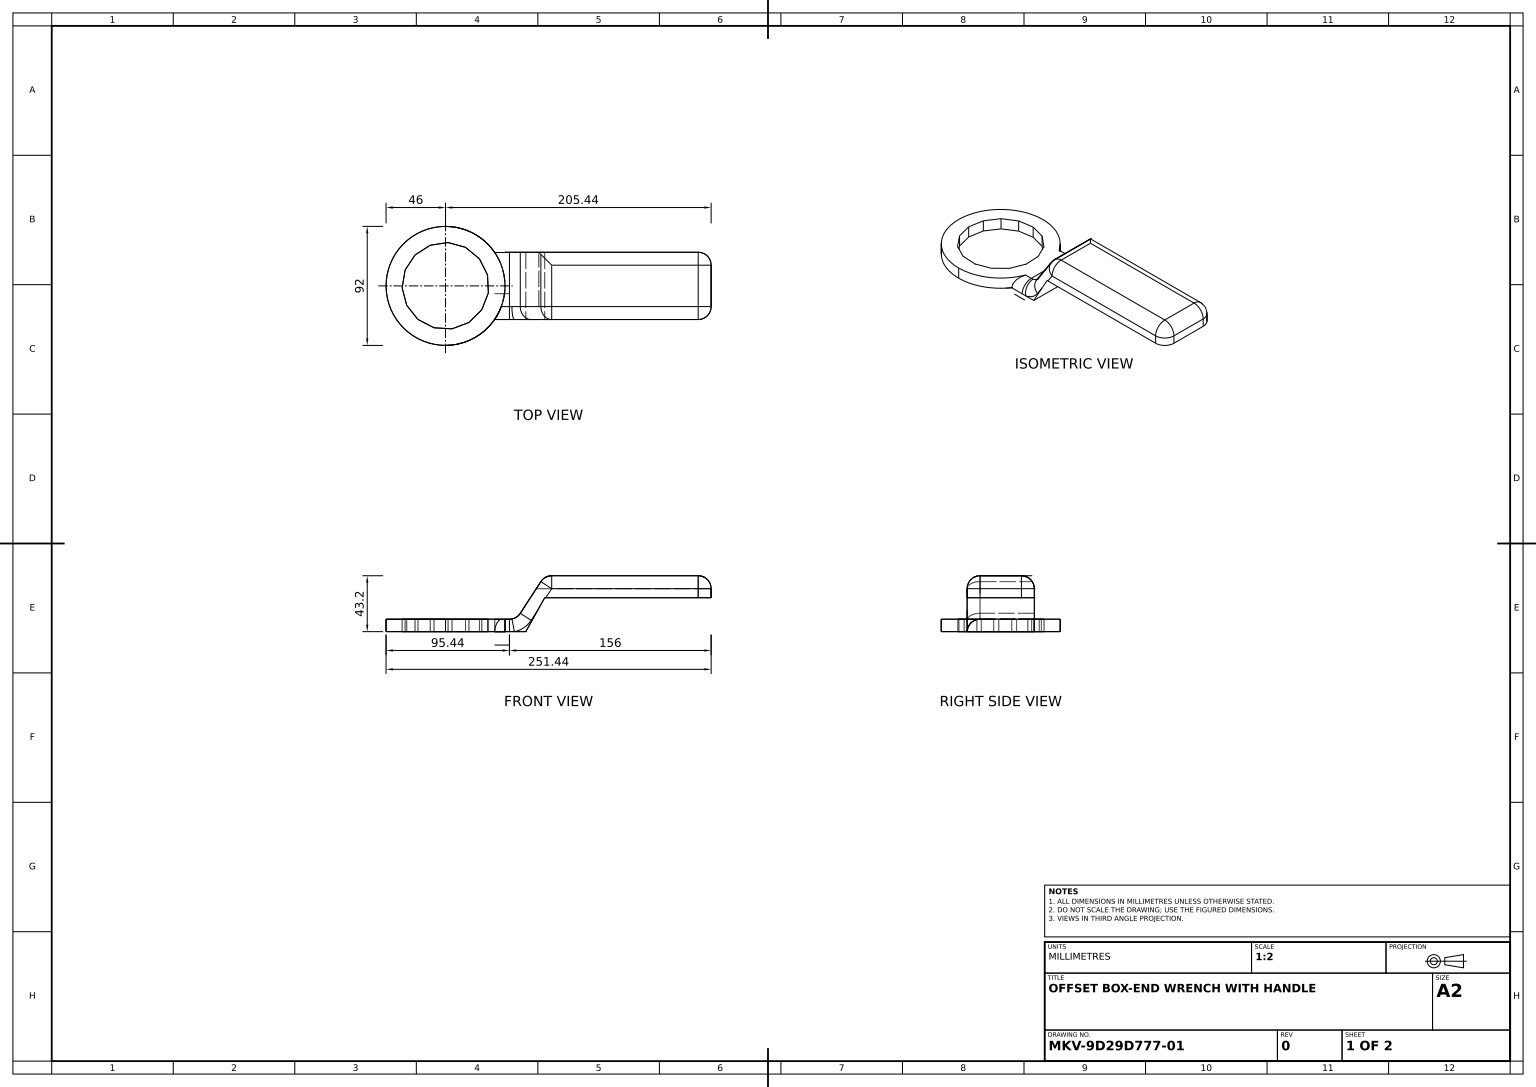
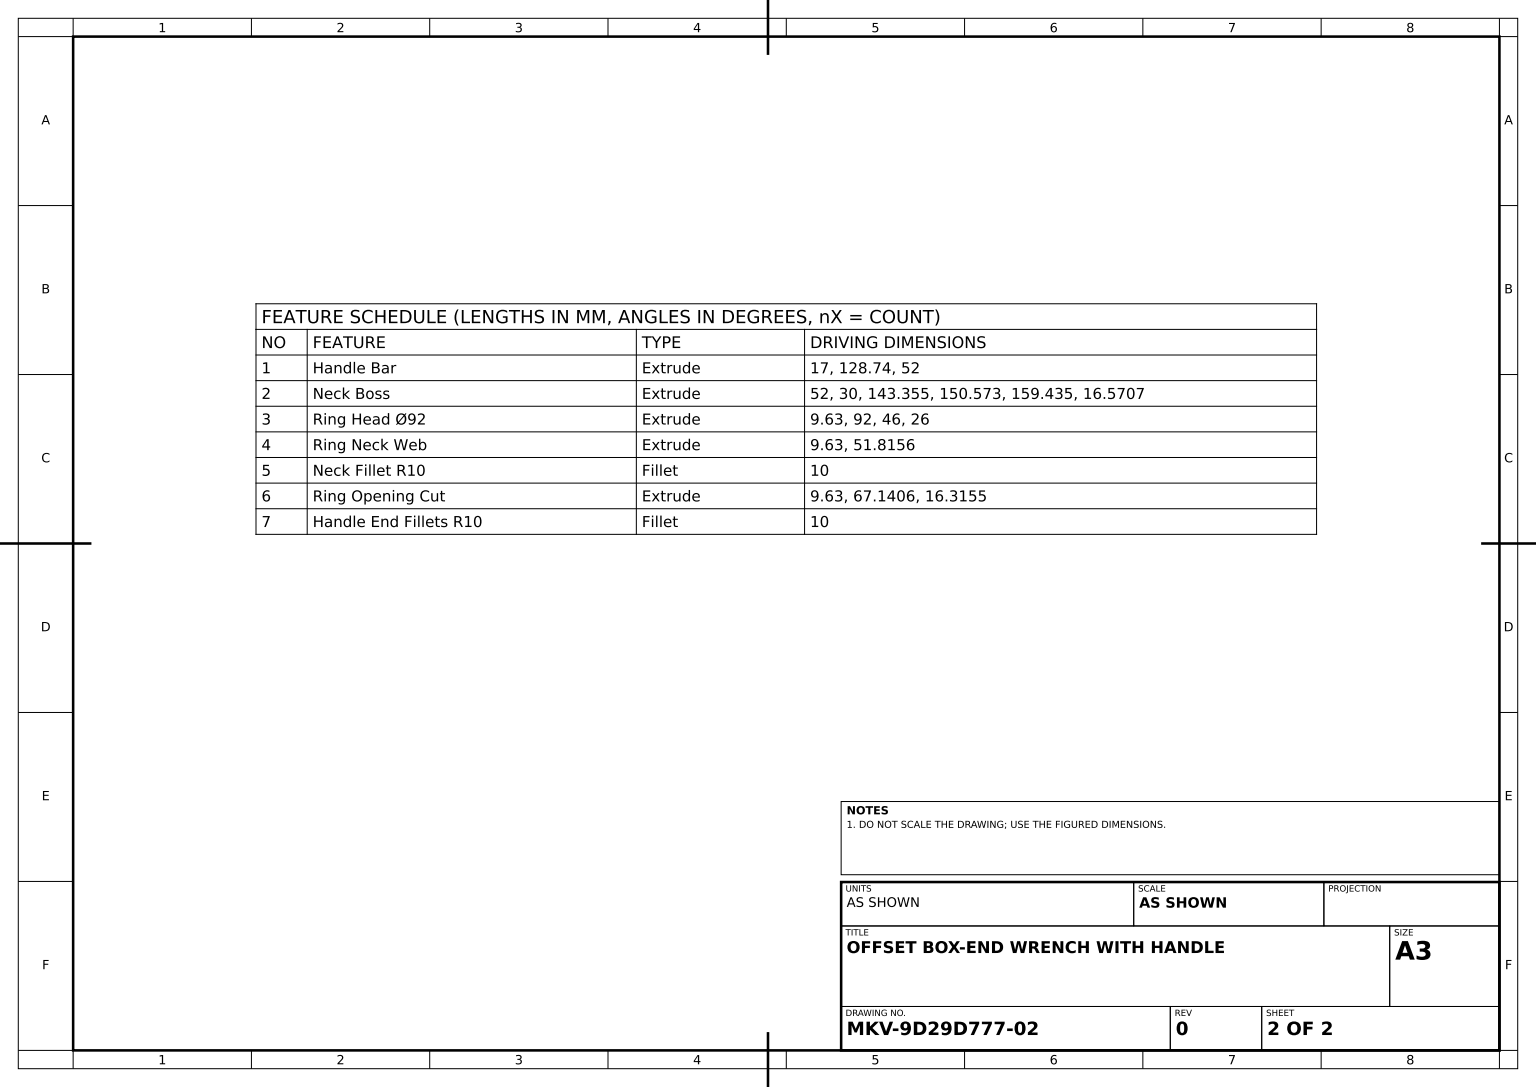
ISO-10303-21;
HEADER;
FILE_DESCRIPTION((''),'2;1');
FILE_NAME('','',(''),(''),'','','');
FILE_SCHEMA(('AUTOMOTIVE_DESIGN'));
ENDSEC;
DATA;
#1=APPLICATION_CONTEXT('');
#2=PRODUCT_CONTEXT('',#1,'mechanical');
#3=PRODUCT('','','',(#2));
#4=PRODUCT_DEFINITION_FORMATION('','',#3);
#5=PRODUCT_DEFINITION_CONTEXT('',#1,'design');
#6=PRODUCT_DEFINITION('','',#4,#5);
#7=PRODUCT_DEFINITION_SHAPE('','',#6);
#8=(LENGTH_UNIT()NAMED_UNIT(*)SI_UNIT(.MILLI.,.METRE.));
#9=(NAMED_UNIT(*)PLANE_ANGLE_UNIT()SI_UNIT($,.RADIAN.));
#10=(NAMED_UNIT(*)SI_UNIT($,.STERADIAN.)SOLID_ANGLE_UNIT());
#11=UNCERTAINTY_MEASURE_WITH_UNIT(LENGTH_MEASURE(1.E-05),#8,'distance_accuracy_value','');
#12=(GEOMETRIC_REPRESENTATION_CONTEXT(3)GLOBAL_UNCERTAINTY_ASSIGNED_CONTEXT((#11))GLOBAL_UNIT_ASSIGNED_CONTEXT((#8,#9,#10))REPRESENTATION_CONTEXT('',''));
#13=CARTESIAN_POINT('',(-87.791409,-26.199202,26.));
#14=VERTEX_POINT('',#13);
#15=CARTESIAN_POINT('',(-89.709963,-16.38497,16.));
#16=VERTEX_POINT('',#15);
#17=CARTESIAN_POINT('',(-87.791409,-26.199202,16.));
#18=DIRECTION('',(-0.981423207,-0.191855384,0.));
#19=DIRECTION('',(0.191855384,-0.981423207,0.));
#20=AXIS2_PLACEMENT_3D('',#17,#18,#19);
#21=CIRCLE('',#20,10.);
#22=EDGE_CURVE('',#14,#16,#21,.T.);
#23=ORIENTED_EDGE('',*,*,#22,.F.);
#24=CARTESIAN_POINT('',(-74.862463,-17.474841,26.));
#25=VERTEX_POINT('',#24);
#26=CARTESIAN_POINT('',(-91.628516,-6.570738,26.));
#27=DIRECTION('',(0.,0.,-1.));
#28=DIRECTION('',(-1.,0.,0.));
#29=AXIS2_PLACEMENT_3D('',#26,#27,#28);
#30=CIRCLE('',#29,20.);
#31=EDGE_CURVE('',#25,#14,#30,.T.);
#32=ORIENTED_EDGE('',*,*,#31,.F.);
#33=CARTESIAN_POINT('',(-83.24549,-12.022789,16.));
#34=VERTEX_POINT('',#33);
#35=CARTESIAN_POINT('',(-74.862463,-17.474841,16.));
#36=DIRECTION('',(-0.545205123,-0.838302674,0.));
#37=DIRECTION('',(0.838302674,-0.545205123,0.));
#38=AXIS2_PLACEMENT_3D('',#35,#36,#37);
#39=CIRCLE('',#38,10.);
#40=EDGE_CURVE('',#25,#34,#39,.T.);
#41=ORIENTED_EDGE('',*,*,#40,.T.);
#42=CARTESIAN_POINT('',(-91.628516,-6.570738,16.));
#43=DIRECTION('',(0.,0.,1.));
#44=AXIS2_PLACEMENT_3D('',#42,#43,#28);
#45=CIRCLE('',#44,10.);
#46=EDGE_CURVE('',#16,#34,#45,.T.);
#47=ORIENTED_EDGE('',*,*,#46,.F.);
#48=EDGE_LOOP('',(#23,#32,#41,#47));
#49=FACE_OUTER_BOUND('',#48,.T.);
#50=AXIS2_PLACEMENT_3D('',#42,#27,#28);
#51=TOROIDAL_SURFACE('',#50,20.,10.);
#52=ADVANCED_FACE('',(#49),#51,.T.);
#53=ORIENTED_EDGE('',*,*,#31,.T.);
#54=CARTESIAN_POINT('',(-78.985122,-26.199202,26.));
#55=VERTEX_POINT('',#54);
#56=CARTESIAN_POINT('',(0.,-26.199202,26.));
#57=DIRECTION('',(1.,0.,0.));
#58=VECTOR('',#57,1000.);
#59=LINE('',#56,#58);
#60=EDGE_CURVE('',#14,#55,#59,.T.);
#61=ORIENTED_EDGE('',*,*,#60,.T.);
#62=CARTESIAN_POINT('',(-69.631281,-9.43142,26.));
#63=VERTEX_POINT('',#62);
#64=CARTESIAN_POINT('',(-49.092725,27.386184,26.));
#65=DIRECTION('',(-0.487170738,-0.873306745,0.));
#66=VECTOR('',#65,1000.);
#67=LINE('',#64,#66);
#68=EDGE_CURVE('',#63,#55,#67,.T.);
#69=ORIENTED_EDGE('',*,*,#68,.F.);
#70=VECTOR('',#36,1000.);
#71=LINE('',#24,#70);
#72=EDGE_CURVE('',#63,#25,#71,.T.);
#73=ORIENTED_EDGE('',*,*,#72,.T.);
#74=EDGE_LOOP('',(#53,#61,#69,#73));
#75=FACE_OUTER_BOUND('',#74,.T.);
#76=CARTESIAN_POINT('',(-64.37,17.,26.));
#77=AXIS2_PLACEMENT_3D('',#76,#27,#28);
#78=PLANE('',#77);
#79=ADVANCED_FACE('',(#75),#78,.F.);
#80=CARTESIAN_POINT('',(-172.324486,-26.200738,-12.239874));
#81=VERTEX_POINT('',#80);
#82=CARTESIAN_POINT('',(-172.324486,-16.570738,-12.239874));
#83=VERTEX_POINT('',#82);
#84=DIRECTION('',(0.,1.,0.));
#85=VECTOR('',#84,1000.);
#86=LINE('',#80,#85);
#87=EDGE_CURVE('',#81,#83,#86,.T.);
#88=ORIENTED_EDGE('',*,*,#87,.T.);
#89=CARTESIAN_POINT('',(-174.600375,-16.570738,1.53266));
#90=VERTEX_POINT('',#89);
#91=DIRECTION('',(-0.163037326,0.,0.986619902));
#92=VECTOR('',#91,1000.);
#93=LINE('',#82,#92);
#94=EDGE_CURVE('',#83,#90,#93,.T.);
#95=ORIENTED_EDGE('',*,*,#94,.T.);
#96=CARTESIAN_POINT('',(-174.600375,-26.200738,1.53266));
#97=VERTEX_POINT('',#96);
#98=LINE('',#96,#85);
#99=EDGE_CURVE('',#97,#90,#98,.T.);
#100=ORIENTED_EDGE('',*,*,#99,.F.);
#101=LINE('',#80,#92);
#102=EDGE_CURVE('',#81,#97,#101,.T.);
#103=ORIENTED_EDGE('',*,*,#102,.F.);
#104=EDGE_LOOP('',(#88,#95,#100,#103));
#105=FACE_OUTER_BOUND('',#104,.T.);
#106=DIRECTION('',(-0.986619902,0.,-0.163037326));
#107=AXIS2_PLACEMENT_3D('',#80,#106,#91);
#108=PLANE('',#107);
#109=ADVANCED_FACE('',(#105),#108,.F.);
#110=CARTESIAN_POINT('',(-141.065092,-26.200738,-46.));
#111=VERTEX_POINT('',#110);
#112=CARTESIAN_POINT('',(-141.065092,-16.570738,-46.));
#113=VERTEX_POINT('',#112);
#114=LINE('',#110,#85);
#115=EDGE_CURVE('',#111,#113,#114,.T.);
#116=ORIENTED_EDGE('',*,*,#115,.F.);
#117=CARTESIAN_POINT('',(-141.065092,-26.200738,46.));
#118=VERTEX_POINT('',#117);
#119=CARTESIAN_POINT('',(-141.065092,-26.200738,0.));
#120=AXIS2_PLACEMENT_3D('',#119,#84,#43);
#121=CIRCLE('',#120,46.);
#122=EDGE_CURVE('',#111,#118,#121,.T.);
#123=ORIENTED_EDGE('',*,*,#122,.T.);
#124=CARTESIAN_POINT('',(-141.065092,-16.570738,46.));
#125=VERTEX_POINT('',#124);
#126=LINE('',#117,#85);
#127=EDGE_CURVE('',#118,#125,#126,.T.);
#128=ORIENTED_EDGE('',*,*,#127,.T.);
#129=CARTESIAN_POINT('',(-141.065092,-16.570738,0.));
#130=AXIS2_PLACEMENT_3D('',#129,#84,#43);
#131=CIRCLE('',#130,46.);
#132=EDGE_CURVE('',#113,#125,#131,.T.);
#133=ORIENTED_EDGE('',*,*,#132,.F.);
#134=EDGE_LOOP('',(#116,#123,#128,#133));
#135=FACE_OUTER_BOUND('',#134,.T.);
#136=CYLINDRICAL_SURFACE('',#120,46.);
#137=ADVANCED_FACE('',(#135),#136,.T.);
#138=CARTESIAN_POINT('',(-122.970128,-16.570738,28.276077));
#139=VERTEX_POINT('',#138);
#140=CARTESIAN_POINT('',(-113.033603,-16.570738,18.471597));
#141=VERTEX_POINT('',#140);
#142=DIRECTION('',(0.711820595,0.,-0.702361332));
#143=VECTOR('',#142,1000.);
#144=LINE('',#138,#143);
#145=EDGE_CURVE('',#139,#141,#144,.T.);
#146=ORIENTED_EDGE('',*,*,#145,.T.);
#147=CARTESIAN_POINT('',(-113.033603,-26.200738,18.471597));
#148=VERTEX_POINT('',#147);
#149=LINE('',#147,#85);
#150=EDGE_CURVE('',#148,#141,#149,.T.);
#151=ORIENTED_EDGE('',*,*,#150,.F.);
#152=CARTESIAN_POINT('',(-122.970128,-26.200738,28.276077));
#153=VERTEX_POINT('',#152);
#154=LINE('',#152,#143);
#155=EDGE_CURVE('',#153,#148,#154,.T.);
#156=ORIENTED_EDGE('',*,*,#155,.F.);
#157=LINE('',#152,#85);
#158=EDGE_CURVE('',#153,#139,#157,.T.);
#159=ORIENTED_EDGE('',*,*,#158,.T.);
#160=EDGE_LOOP('',(#146,#151,#156,#159));
#161=FACE_OUTER_BOUND('',#160,.T.);
#162=DIRECTION('',(0.702361332,0.,0.711820595));
#163=AXIS2_PLACEMENT_3D('',#152,#162,#142);
#164=PLANE('',#163);
#165=ADVANCED_FACE('',(#161),#164,.F.);
#166=CARTESIAN_POINT('',(-136.035437,-26.200738,33.191367));
#167=VERTEX_POINT('',#166);
#168=DIRECTION('',(0.935956562,0.,-0.352115485));
#169=VECTOR('',#168,1000.);
#170=LINE('',#166,#169);
#171=EDGE_CURVE('',#167,#153,#170,.T.);
#172=ORIENTED_EDGE('',*,*,#171,.F.);
#173=CARTESIAN_POINT('',(-136.035437,-16.570738,33.191367));
#174=VERTEX_POINT('',#173);
#175=LINE('',#166,#85);
#176=EDGE_CURVE('',#167,#174,#175,.T.);
#177=ORIENTED_EDGE('',*,*,#176,.T.);
#178=LINE('',#173,#169);
#179=EDGE_CURVE('',#174,#139,#178,.T.);
#180=ORIENTED_EDGE('',*,*,#179,.T.);
#181=ORIENTED_EDGE('',*,*,#158,.F.);
#182=EDGE_LOOP('',(#172,#177,#180,#181));
#183=FACE_OUTER_BOUND('',#182,.T.);
#184=DIRECTION('',(0.352115485,0.,0.935956562));
#185=AXIS2_PLACEMENT_3D('',#166,#184,#168);
#186=PLANE('',#185);
#187=ADVANCED_FACE('',(#183),#186,.F.);
#188=CARTESIAN_POINT('',(-107.943977,-16.570738,5.47321));
#189=VERTEX_POINT('',#188);
#190=CARTESIAN_POINT('',(-108.581293,-16.570738,-8.471545));
#191=VERTEX_POINT('',#190);
#192=DIRECTION('',(-0.045655243,0.,-0.998957256));
#193=VECTOR('',#192,1000.);
#194=LINE('',#188,#193);
#195=EDGE_CURVE('',#189,#191,#194,.T.);
#196=ORIENTED_EDGE('',*,*,#195,.T.);
#197=CARTESIAN_POINT('',(-108.581293,-26.200738,-8.471545));
#198=VERTEX_POINT('',#197);
#199=LINE('',#197,#85);
#200=EDGE_CURVE('',#198,#191,#199,.T.);
#201=ORIENTED_EDGE('',*,*,#200,.F.);
#202=CARTESIAN_POINT('',(-107.943977,-26.200738,5.47321));
#203=VERTEX_POINT('',#202);
#204=LINE('',#202,#193);
#205=EDGE_CURVE('',#203,#198,#204,.T.);
#206=ORIENTED_EDGE('',*,*,#205,.F.);
#207=LINE('',#202,#85);
#208=EDGE_CURVE('',#203,#189,#207,.T.);
#209=ORIENTED_EDGE('',*,*,#208,.T.);
#210=EDGE_LOOP('',(#196,#201,#206,#209));
#211=FACE_OUTER_BOUND('',#210,.T.);
#212=DIRECTION('',(0.998957256,0.,-0.045655243));
#213=AXIS2_PLACEMENT_3D('',#202,#212,#192);
#214=PLANE('',#213);
#215=ADVANCED_FACE('',(#211),#214,.F.);
#216=ORIENTED_EDGE('',*,*,#102,.T.);
#217=CARTESIAN_POINT('',(-171.077709,-26.200738,15.040183));
#218=VERTEX_POINT('',#217);
#219=DIRECTION('',(0.252352458,0.,0.967635384));
#220=VECTOR('',#219,1000.);
#221=LINE('',#96,#220);
#222=EDGE_CURVE('',#97,#218,#221,.T.);
#223=ORIENTED_EDGE('',*,*,#222,.T.);
#224=CARTESIAN_POINT('',(-162.365588,-26.200738,25.947122));
#225=VERTEX_POINT('',#224);
#226=DIRECTION('',(0.62410821,0.,0.781337918));
#227=VECTOR('',#226,1000.);
#228=LINE('',#217,#227);
#229=EDGE_CURVE('',#218,#225,#228,.T.);
#230=ORIENTED_EDGE('',*,*,#229,.T.);
#231=CARTESIAN_POINT('',(-149.970418,-26.200738,32.367567));
#232=VERTEX_POINT('',#231);
#233=DIRECTION('',(0.887949982,0.,0.459940028));
#234=VECTOR('',#233,1000.);
#235=LINE('',#224,#234);
#236=EDGE_CURVE('',#225,#232,#235,.T.);
#237=ORIENTED_EDGE('',*,*,#236,.T.);
#238=DIRECTION('',(0.998257136,0.,0.059014328));
#239=VECTOR('',#238,1000.);
#240=LINE('',#231,#239);
#241=EDGE_CURVE('',#232,#167,#240,.T.);
#242=ORIENTED_EDGE('',*,*,#241,.T.);
#243=ORIENTED_EDGE('',*,*,#171,.T.);
#244=ORIENTED_EDGE('',*,*,#155,.T.);
#245=DIRECTION('',(0.364604381,0.,-0.931162524));
#246=VECTOR('',#245,1000.);
#247=LINE('',#147,#246);
#248=EDGE_CURVE('',#148,#203,#247,.T.);
#249=ORIENTED_EDGE('',*,*,#248,.T.);
#250=ORIENTED_EDGE('',*,*,#205,.T.);
#251=CARTESIAN_POINT('',(-114.835353,-26.200738,-20.951493));
#252=VERTEX_POINT('',#251);
#253=DIRECTION('',(-0.448020661,0.,-0.894023203));
#254=VECTOR('',#253,1000.);
#255=LINE('',#197,#254);
#256=EDGE_CURVE('',#198,#252,#255,.T.);
#257=ORIENTED_EDGE('',*,*,#256,.T.);
#258=CARTESIAN_POINT('',(-125.624772,-26.200738,-29.808737));
#259=VERTEX_POINT('',#258);
#260=DIRECTION('',(-0.772919236,0.,-0.634504417));
#261=VECTOR('',#260,1000.);
#262=LINE('',#251,#261);
#263=EDGE_CURVE('',#252,#259,#262,.T.);
#264=ORIENTED_EDGE('',*,*,#263,.T.);
#265=CARTESIAN_POINT('',(-139.083964,-26.200738,-33.51178));
#266=VERTEX_POINT('',#265);
#267=DIRECTION('',(-0.964173054,0.,-0.265274052));
#268=VECTOR('',#267,1000.);
#269=LINE('',#258,#268);
#270=EDGE_CURVE('',#259,#266,#269,.T.);
#271=ORIENTED_EDGE('',*,*,#270,.T.);
#272=CARTESIAN_POINT('',(-152.88571,-26.200738,-31.420332));
#273=VERTEX_POINT('',#272);
#274=DIRECTION('',(-0.988712591,0.,0.149824606));
#275=VECTOR('',#274,1000.);
#276=LINE('',#265,#275);
#277=EDGE_CURVE('',#266,#273,#276,.T.);
#278=ORIENTED_EDGE('',*,*,#277,.T.);
#279=CARTESIAN_POINT('',(-164.643564,-26.200738,-23.896023));
#280=VERTEX_POINT('',#279);
#281=DIRECTION('',(-0.842294739,0.,0.539017228));
#282=VECTOR('',#281,1000.);
#283=LINE('',#272,#282);
#284=EDGE_CURVE('',#273,#280,#283,.T.);
#285=ORIENTED_EDGE('',*,*,#284,.T.);
#286=DIRECTION('',(-0.550236475,0.,0.835008875));
#287=VECTOR('',#286,1000.);
#288=LINE('',#279,#287);
#289=EDGE_CURVE('',#280,#81,#288,.T.);
#290=ORIENTED_EDGE('',*,*,#289,.T.);
#291=EDGE_LOOP('',(#216,#223,#230,#237,#242,#243,#244,#249,#250,#257,#264,#271,#278,#285,#290));
#292=FACE_BOUND('',#291,.T.);
#293=EDGE_CURVE('',#118,#111,#121,.T.);
#294=ORIENTED_EDGE('',*,*,#293,.F.);
#295=ORIENTED_EDGE('',*,*,#122,.F.);
#296=EDGE_LOOP('',(#294,#295));
#297=FACE_OUTER_BOUND('',#296,.T.);
#298=PLANE('',#120);
#299=ADVANCED_FACE('',(#292,#297),#298,.F.);
#300=CARTESIAN_POINT('',(-152.88571,-16.570738,-31.420332));
#301=VERTEX_POINT('',#300);
#302=LINE('',#272,#85);
#303=EDGE_CURVE('',#273,#301,#302,.T.);
#304=ORIENTED_EDGE('',*,*,#303,.F.);
#305=ORIENTED_EDGE('',*,*,#277,.F.);
#306=CARTESIAN_POINT('',(-139.083964,-16.570738,-33.51178));
#307=VERTEX_POINT('',#306);
#308=LINE('',#265,#85);
#309=EDGE_CURVE('',#266,#307,#308,.T.);
#310=ORIENTED_EDGE('',*,*,#309,.T.);
#311=LINE('',#306,#275);
#312=EDGE_CURVE('',#307,#301,#311,.T.);
#313=ORIENTED_EDGE('',*,*,#312,.T.);
#314=EDGE_LOOP('',(#304,#305,#310,#313));
#315=FACE_OUTER_BOUND('',#314,.T.);
#316=DIRECTION('',(-0.149824606,0.,-0.988712591));
#317=AXIS2_PLACEMENT_3D('',#265,#316,#274);
#318=PLANE('',#317);
#319=ADVANCED_FACE('',(#315),#318,.F.);
#320=CARTESIAN_POINT('',(64.37,7.,16.));
#321=VERTEX_POINT('',#320);
#322=CARTESIAN_POINT('',(54.37,17.,16.));
#323=VERTEX_POINT('',#322);
#324=CARTESIAN_POINT('',(54.37,7.,16.));
#325=AXIS2_PLACEMENT_3D('',#324,#43,#57);
#326=CIRCLE('',#325,10.);
#327=EDGE_CURVE('',#321,#323,#326,.T.);
#328=ORIENTED_EDGE('',*,*,#327,.T.);
#329=CARTESIAN_POINT('',(54.37,7.,26.));
#330=VERTEX_POINT('',#329);
#331=AXIS2_PLACEMENT_3D('',#324,#28,#27);
#332=CIRCLE('',#331,10.);
#333=EDGE_CURVE('',#330,#323,#332,.T.);
#334=ORIENTED_EDGE('',*,*,#333,.F.);
#335=AXIS2_PLACEMENT_3D('',#324,#84,#43);
#336=CIRCLE('',#335,10.);
#337=EDGE_CURVE('',#330,#321,#336,.T.);
#338=ORIENTED_EDGE('',*,*,#337,.T.);
#339=EDGE_LOOP('',(#328,#334,#338));
#340=FACE_OUTER_BOUND('',#339,.T.);
#341=AXIS2_PLACEMENT_3D('',#324,#84,#57);
#342=SPHERICAL_SURFACE('',#341,10.);
#343=ADVANCED_FACE('',(#340),#342,.T.);
#344=ORIENTED_EDGE('',*,*,#208,.F.);
#345=ORIENTED_EDGE('',*,*,#248,.F.);
#346=ORIENTED_EDGE('',*,*,#150,.T.);
#347=LINE('',#140,#246);
#348=EDGE_CURVE('',#141,#189,#347,.T.);
#349=ORIENTED_EDGE('',*,*,#348,.T.);
#350=EDGE_LOOP('',(#344,#345,#346,#349));
#351=FACE_OUTER_BOUND('',#350,.T.);
#352=DIRECTION('',(0.931162524,0.,0.364604381));
#353=AXIS2_PLACEMENT_3D('',#147,#352,#245);
#354=PLANE('',#353);
#355=ADVANCED_FACE('',(#351),#354,.F.);
#356=CARTESIAN_POINT('',(-114.835353,-16.570738,-20.951493));
#357=VERTEX_POINT('',#356);
#358=LINE('',#251,#85);
#359=EDGE_CURVE('',#252,#357,#358,.T.);
#360=ORIENTED_EDGE('',*,*,#359,.F.);
#361=ORIENTED_EDGE('',*,*,#256,.F.);
#362=ORIENTED_EDGE('',*,*,#200,.T.);
#363=LINE('',#190,#254);
#364=EDGE_CURVE('',#191,#357,#363,.T.);
#365=ORIENTED_EDGE('',*,*,#364,.T.);
#366=EDGE_LOOP('',(#360,#361,#362,#365));
#367=FACE_OUTER_BOUND('',#366,.T.);
#368=DIRECTION('',(0.894023203,0.,-0.448020661));
#369=AXIS2_PLACEMENT_3D('',#197,#368,#253);
#370=PLANE('',#369);
#371=ADVANCED_FACE('',(#367),#370,.F.);
#372=CARTESIAN_POINT('',(64.37,0.,16.));
#373=VERTEX_POINT('',#372);
#374=CARTESIAN_POINT('',(54.37,0.,26.));
#375=VERTEX_POINT('',#374);
#376=CARTESIAN_POINT('',(54.37,0.,16.));
#377=DIRECTION('',(0.,-1.,0.));
#378=AXIS2_PLACEMENT_3D('',#376,#377,#27);
#379=CIRCLE('',#378,10.);
#380=EDGE_CURVE('',#373,#375,#379,.T.);
#381=ORIENTED_EDGE('',*,*,#380,.F.);
#382=CARTESIAN_POINT('',(64.37,17.,16.));
#383=VECTOR('',#377,1000.);
#384=LINE('',#382,#383);
#385=EDGE_CURVE('',#321,#373,#384,.T.);
#386=ORIENTED_EDGE('',*,*,#385,.F.);
#387=ORIENTED_EDGE('',*,*,#337,.F.);
#388=CARTESIAN_POINT('',(54.37,17.,26.));
#389=LINE('',#388,#85);
#390=EDGE_CURVE('',#375,#330,#389,.T.);
#391=ORIENTED_EDGE('',*,*,#390,.F.);
#392=EDGE_LOOP('',(#381,#386,#387,#391));
#393=FACE_OUTER_BOUND('',#392,.T.);
#394=AXIS2_PLACEMENT_3D('',#322,#377,#27);
#395=CYLINDRICAL_SURFACE('',#394,10.);
#396=ADVANCED_FACE('',(#393),#395,.T.);
#397=CARTESIAN_POINT('',(-91.628516,-16.570738,-26.));
#398=VERTEX_POINT('',#397);
#399=CARTESIAN_POINT('',(-95.065092,-16.570738,-26.));
#400=VERTEX_POINT('',#399);
#401=CARTESIAN_POINT('',(0.,-16.570738,-26.));
#402=VECTOR('',#28,1000.);
#403=LINE('',#401,#402);
#404=EDGE_CURVE('',#398,#400,#403,.T.);
#405=ORIENTED_EDGE('',*,*,#404,.T.);
#406=CARTESIAN_POINT('',(-95.065092,-16.570738,-25.815581));
#407=VERTEX_POINT('',#406);
#408=VECTOR('',#43,1000.);
#409=LINE('',#399,#408);
#410=EDGE_CURVE('',#400,#407,#409,.T.);
#411=ORIENTED_EDGE('',*,*,#410,.T.);
#412=CARTESIAN_POINT('',(-102.99206,-16.570738,-25.815581));
#413=VERTEX_POINT('',#412);
#414=CARTESIAN_POINT('',(-104.695092,-16.570738,-25.815581));
#415=LINE('',#414,#58);
#416=EDGE_CURVE('',#413,#407,#415,.T.);
#417=ORIENTED_EDGE('',*,*,#416,.F.);
#418=EDGE_CURVE('',#413,#113,#131,.T.);
#419=ORIENTED_EDGE('',*,*,#418,.T.);
#420=ORIENTED_EDGE('',*,*,#132,.T.);
#421=CARTESIAN_POINT('',(-97.939937,-16.570738,16.006904));
#422=VERTEX_POINT('',#421);
#423=EDGE_CURVE('',#125,#422,#131,.T.);
#424=ORIENTED_EDGE('',*,*,#423,.T.);
#425=CARTESIAN_POINT('',(-91.628516,-16.570738,16.006904));
#426=VERTEX_POINT('',#425);
#427=LINE('',#425,#58);
#428=EDGE_CURVE('',#422,#426,#427,.T.);
#429=ORIENTED_EDGE('',*,*,#428,.T.);
#430=VECTOR('',#27,1000.);
#431=LINE('',#397,#430);
#432=EDGE_CURVE('',#426,#398,#431,.T.);
#433=ORIENTED_EDGE('',*,*,#432,.T.);
#434=EDGE_LOOP('',(#405,#411,#417,#419,#420,#424,#429,#433));
#435=FACE_OUTER_BOUND('',#434,.T.);
#436=ORIENTED_EDGE('',*,*,#145,.F.);
#437=ORIENTED_EDGE('',*,*,#179,.F.);
#438=CARTESIAN_POINT('',(-149.970418,-16.570738,32.367567));
#439=VERTEX_POINT('',#438);
#440=LINE('',#438,#239);
#441=EDGE_CURVE('',#439,#174,#440,.T.);
#442=ORIENTED_EDGE('',*,*,#441,.F.);
#443=CARTESIAN_POINT('',(-162.365588,-16.570738,25.947122));
#444=VERTEX_POINT('',#443);
#445=LINE('',#443,#234);
#446=EDGE_CURVE('',#444,#439,#445,.T.);
#447=ORIENTED_EDGE('',*,*,#446,.F.);
#448=CARTESIAN_POINT('',(-171.077709,-16.570738,15.040183));
#449=VERTEX_POINT('',#448);
#450=LINE('',#448,#227);
#451=EDGE_CURVE('',#449,#444,#450,.T.);
#452=ORIENTED_EDGE('',*,*,#451,.F.);
#453=LINE('',#89,#220);
#454=EDGE_CURVE('',#90,#449,#453,.T.);
#455=ORIENTED_EDGE('',*,*,#454,.F.);
#456=ORIENTED_EDGE('',*,*,#94,.F.);
#457=CARTESIAN_POINT('',(-164.643564,-16.570738,-23.896023));
#458=VERTEX_POINT('',#457);
#459=LINE('',#457,#287);
#460=EDGE_CURVE('',#458,#83,#459,.T.);
#461=ORIENTED_EDGE('',*,*,#460,.F.);
#462=LINE('',#300,#282);
#463=EDGE_CURVE('',#301,#458,#462,.T.);
#464=ORIENTED_EDGE('',*,*,#463,.F.);
#465=ORIENTED_EDGE('',*,*,#312,.F.);
#466=CARTESIAN_POINT('',(-125.624772,-16.570738,-29.808737));
#467=VERTEX_POINT('',#466);
#468=LINE('',#466,#268);
#469=EDGE_CURVE('',#467,#307,#468,.T.);
#470=ORIENTED_EDGE('',*,*,#469,.F.);
#471=LINE('',#356,#261);
#472=EDGE_CURVE('',#357,#467,#471,.T.);
#473=ORIENTED_EDGE('',*,*,#472,.F.);
#474=ORIENTED_EDGE('',*,*,#364,.F.);
#475=ORIENTED_EDGE('',*,*,#195,.F.);
#476=ORIENTED_EDGE('',*,*,#348,.F.);
#477=EDGE_LOOP('',(#436,#437,#442,#447,#452,#455,#456,#461,#464,#465,#470,#473,#474,#475,#476));
#478=FACE_BOUND('',#477,.T.);
#479=AXIS2_PLACEMENT_3D('',#401,#84,#43);
#480=PLANE('',#479);
#481=ADVANCED_FACE('',(#435,#478),#480,.T.);
#482=CARTESIAN_POINT('',(-95.065092,-26.199202,-26.));
#483=VERTEX_POINT('',#482);
#484=CARTESIAN_POINT('',(-95.065092,-26.199202,-25.815581));
#485=VERTEX_POINT('',#484);
#486=LINE('',#482,#408);
#487=EDGE_CURVE('',#483,#485,#486,.T.);
#488=ORIENTED_EDGE('',*,*,#487,.T.);
#489=LINE('',#406,#383);
#490=EDGE_CURVE('',#407,#485,#489,.T.);
#491=ORIENTED_EDGE('',*,*,#490,.F.);
#492=ORIENTED_EDGE('',*,*,#410,.F.);
#493=CARTESIAN_POINT('',(-95.065092,0.,-26.));
#494=LINE('',#493,#383);
#495=EDGE_CURVE('',#400,#483,#494,.T.);
#496=ORIENTED_EDGE('',*,*,#495,.T.);
#497=EDGE_LOOP('',(#488,#491,#492,#496));
#498=FACE_OUTER_BOUND('',#497,.T.);
#499=AXIS2_PLACEMENT_3D('',#493,#28,#43);
#500=PLANE('',#499);
#501=ADVANCED_FACE('',(#498),#500,.T.);
#502=ORIENTED_EDGE('',*,*,#68,.T.);
#503=CARTESIAN_POINT('',(-78.985122,-26.199202,-26.));
#504=VERTEX_POINT('',#503);
#505=LINE('',#503,#408);
#506=EDGE_CURVE('',#504,#55,#505,.T.);
#507=ORIENTED_EDGE('',*,*,#506,.F.);
#508=CARTESIAN_POINT('',(-64.37,0.,-26.));
#509=VERTEX_POINT('',#508);
#510=CARTESIAN_POINT('',(-49.092725,27.386184,-26.));
#511=LINE('',#510,#66);
#512=EDGE_CURVE('',#509,#504,#511,.T.);
#513=ORIENTED_EDGE('',*,*,#512,.F.);
#514=CARTESIAN_POINT('',(-64.37,0.,25.973209));
#515=VERTEX_POINT('',#514);
#516=CARTESIAN_POINT('',(-64.37,0.,26.));
#517=LINE('',#516,#408);
#518=EDGE_CURVE('',#509,#515,#517,.T.);
#519=ORIENTED_EDGE('',*,*,#518,.T.);
#520=CARTESIAN_POINT('',(-66.121016,-3.138888,25.991066));
#521=CARTESIAN_POINT('',(-67.87556,-6.2841,26.));
#522=(BOUNDED_CURVE()B_SPLINE_CURVE(3,(#514,#520,#521,#62),.UNSPECIFIED.,.F.,.T.)B_SPLINE_CURVE_WITH_KNOTS((4,4),(1.497579638,1.570796327),.UNSPECIFIED.)CURVE()GEOMETRIC_REPRESENTATION_ITEM()RATIONAL_B_SPLINE_CURVE((1.,0.999553326,0.999553326,1.))REPRESENTATION_ITEM(''));
#523=EDGE_CURVE('',#515,#63,#522,.T.);
#524=ORIENTED_EDGE('',*,*,#523,.T.);
#525=EDGE_LOOP('',(#502,#507,#513,#519,#524));
#526=FACE_OUTER_BOUND('',#525,.T.);
#527=DIRECTION('',(-0.873306745,0.487170738,0.));
#528=AXIS2_PLACEMENT_3D('',#510,#527,#65);
#529=PLANE('',#528);
#530=ADVANCED_FACE('',(#526),#529,.F.);
#531=CARTESIAN_POINT('',(64.37,7.,-16.));
#532=VERTEX_POINT('',#531);
#533=CARTESIAN_POINT('',(54.37,17.,-16.));
#534=VERTEX_POINT('',#533);
#535=CARTESIAN_POINT('',(54.37,7.,-16.));
#536=AXIS2_PLACEMENT_3D('',#535,#43,#28);
#537=CIRCLE('',#536,10.);
#538=EDGE_CURVE('',#532,#534,#537,.T.);
#539=ORIENTED_EDGE('',*,*,#538,.F.);
#540=CARTESIAN_POINT('',(54.37,7.,-26.));
#541=VERTEX_POINT('',#540);
#542=AXIS2_PLACEMENT_3D('',#535,#84,#43);
#543=CIRCLE('',#542,10.);
#544=EDGE_CURVE('',#532,#541,#543,.T.);
#545=ORIENTED_EDGE('',*,*,#544,.T.);
#546=AXIS2_PLACEMENT_3D('',#535,#28,#84);
#547=CIRCLE('',#546,10.);
#548=EDGE_CURVE('',#534,#541,#547,.T.);
#549=ORIENTED_EDGE('',*,*,#548,.F.);
#550=EDGE_LOOP('',(#539,#545,#549));
#551=FACE_OUTER_BOUND('',#550,.T.);
#552=AXIS2_PLACEMENT_3D('',#535,#84,#57);
#553=SPHERICAL_SURFACE('',#552,10.);
#554=ADVANCED_FACE('',(#551),#553,.T.);
#555=ORIENTED_EDGE('',*,*,#446,.T.);
#556=LINE('',#231,#85);
#557=EDGE_CURVE('',#232,#439,#556,.T.);
#558=ORIENTED_EDGE('',*,*,#557,.F.);
#559=ORIENTED_EDGE('',*,*,#236,.F.);
#560=LINE('',#224,#85);
#561=EDGE_CURVE('',#225,#444,#560,.T.);
#562=ORIENTED_EDGE('',*,*,#561,.T.);
#563=EDGE_LOOP('',(#555,#558,#559,#562));
#564=FACE_OUTER_BOUND('',#563,.T.);
#565=DIRECTION('',(-0.459940028,0.,0.887949982));
#566=AXIS2_PLACEMENT_3D('',#224,#565,#233);
#567=PLANE('',#566);
#568=ADVANCED_FACE('',(#564),#567,.F.);
#569=CARTESIAN_POINT('',(-83.24549,-12.022789,-26.));
#570=VERTEX_POINT('',#569);
#571=CARTESIAN_POINT('',(-83.24549,-12.022789,26.));
#572=LINE('',#571,#408);
#573=EDGE_CURVE('',#570,#34,#572,.T.);
#574=ORIENTED_EDGE('',*,*,#573,.F.);
#575=CARTESIAN_POINT('',(-91.628516,-6.570738,-26.));
#576=AXIS2_PLACEMENT_3D('',#575,#43,#57);
#577=CIRCLE('',#576,10.);
#578=EDGE_CURVE('',#398,#570,#577,.T.);
#579=ORIENTED_EDGE('',*,*,#578,.F.);
#580=ORIENTED_EDGE('',*,*,#432,.F.);
#581=CARTESIAN_POINT('',(-90.982994,-16.570738,16.006904));
#582=CARTESIAN_POINT('',(-90.343493,-16.508817,16.));
#583=B_SPLINE_CURVE_WITH_KNOTS('',3,(#425,#581,#582,#15),.UNSPECIFIED.,.F.,.F.,(4,4),(0.,0.001927539),.UNSPECIFIED.);
#584=EDGE_CURVE('',#426,#16,#583,.T.);
#585=ORIENTED_EDGE('',*,*,#584,.T.);
#586=ORIENTED_EDGE('',*,*,#46,.T.);
#587=EDGE_LOOP('',(#574,#579,#580,#585,#586));
#588=FACE_OUTER_BOUND('',#587,.T.);
#589=AXIS2_PLACEMENT_3D('',#575,#27,#28);
#590=CYLINDRICAL_SURFACE('',#589,10.);
#591=ADVANCED_FACE('',(#588),#590,.F.);
#592=CARTESIAN_POINT('',(-102.99206,-26.199202,-25.815581));
#593=VERTEX_POINT('',#592);
#594=CARTESIAN_POINT('',(-103.11776,-26.199202,26.));
#595=VERTEX_POINT('',#594);
#596=CARTESIAN_POINT('',(-141.065092,-26.199202,0.));
#597=AXIS2_PLACEMENT_3D('',#596,#377,#27);
#598=CIRCLE('',#597,46.);
#599=EDGE_CURVE('',#593,#595,#598,.T.);
#600=ORIENTED_EDGE('',*,*,#599,.F.);
#601=CARTESIAN_POINT('',(-104.695092,-26.199202,-25.815581));
#602=LINE('',#601,#58);
#603=EDGE_CURVE('',#593,#485,#602,.T.);
#604=ORIENTED_EDGE('',*,*,#603,.T.);
#605=ORIENTED_EDGE('',*,*,#487,.F.);
#606=CARTESIAN_POINT('',(0.,-26.199202,-26.));
#607=LINE('',#606,#58);
#608=EDGE_CURVE('',#483,#504,#607,.T.);
#609=ORIENTED_EDGE('',*,*,#608,.T.);
#610=ORIENTED_EDGE('',*,*,#506,.T.);
#611=ORIENTED_EDGE('',*,*,#60,.F.);
#612=CARTESIAN_POINT('',(-91.628516,-26.199202,26.));
#613=VERTEX_POINT('',#612);
#614=EDGE_CURVE('',#613,#14,#59,.T.);
#615=ORIENTED_EDGE('',*,*,#614,.F.);
#616=EDGE_CURVE('',#595,#613,#59,.T.);
#617=ORIENTED_EDGE('',*,*,#616,.F.);
#618=EDGE_LOOP('',(#600,#604,#605,#609,#610,#611,#615,#617));
#619=FACE_OUTER_BOUND('',#618,.T.);
#620=AXIS2_PLACEMENT_3D('',#606,#377,#27);
#621=PLANE('',#620);
#622=ADVANCED_FACE('',(#619),#621,.T.);
#623=ORIENTED_EDGE('',*,*,#99,.T.);
#624=ORIENTED_EDGE('',*,*,#454,.T.);
#625=LINE('',#217,#85);
#626=EDGE_CURVE('',#218,#449,#625,.T.);
#627=ORIENTED_EDGE('',*,*,#626,.F.);
#628=ORIENTED_EDGE('',*,*,#222,.F.);
#629=EDGE_LOOP('',(#623,#624,#627,#628));
#630=FACE_OUTER_BOUND('',#629,.T.);
#631=DIRECTION('',(-0.967635384,0.,0.252352458));
#632=AXIS2_PLACEMENT_3D('',#96,#631,#219);
#633=PLANE('',#632);
#634=ADVANCED_FACE('',(#630),#633,.F.);
#635=ORIENTED_EDGE('',*,*,#469,.T.);
#636=ORIENTED_EDGE('',*,*,#309,.F.);
#637=ORIENTED_EDGE('',*,*,#270,.F.);
#638=LINE('',#258,#85);
#639=EDGE_CURVE('',#259,#467,#638,.T.);
#640=ORIENTED_EDGE('',*,*,#639,.T.);
#641=EDGE_LOOP('',(#635,#636,#637,#640));
#642=FACE_OUTER_BOUND('',#641,.T.);
#643=DIRECTION('',(0.265274052,0.,-0.964173054));
#644=AXIS2_PLACEMENT_3D('',#258,#643,#267);
#645=PLANE('',#644);
#646=ADVANCED_FACE('',(#642),#645,.F.);
#647=CARTESIAN_POINT('',(-58.944813,7.,26.));
#648=VERTEX_POINT('',#647);
#649=CARTESIAN_POINT('',(-58.944813,17.,16.));
#650=VERTEX_POINT('',#649);
#651=CARTESIAN_POINT('',(-58.944813,7.,16.));
#652=AXIS2_PLACEMENT_3D('',#651,#28,#377);
#653=CIRCLE('',#652,10.);
#654=EDGE_CURVE('',#648,#650,#653,.T.);
#655=ORIENTED_EDGE('',*,*,#654,.T.);
#656=CARTESIAN_POINT('',(-67.32784,12.452051,16.));
#657=VERTEX_POINT('',#656);
#658=AXIS2_PLACEMENT_3D('',#651,#43,#57);
#659=CIRCLE('',#658,10.);
#660=EDGE_CURVE('',#650,#657,#659,.T.);
#661=ORIENTED_EDGE('',*,*,#660,.T.);
#662=DIRECTION('',(-0.838302674,0.545205123,0.));
#663=AXIS2_PLACEMENT_3D('',#651,#36,#662);
#664=CIRCLE('',#663,10.);
#665=EDGE_CURVE('',#648,#657,#664,.T.);
#666=ORIENTED_EDGE('',*,*,#665,.F.);
#667=EDGE_LOOP('',(#655,#661,#666));
#668=FACE_OUTER_BOUND('',#667,.T.);
#669=AXIS2_PLACEMENT_3D('',#651,#84,#57);
#670=SPHERICAL_SURFACE('',#669,10.);
#671=ADVANCED_FACE('',(#668),#670,.T.);
#672=ORIENTED_EDGE('',*,*,#573,.T.);
#673=CARTESIAN_POINT('',(-64.37,17.,16.));
#674=DIRECTION('',(0.545205123,0.838302674,0.));
#675=VECTOR('',#674,1000.);
#676=LINE('',#673,#675);
#677=EDGE_CURVE('',#34,#657,#676,.T.);
#678=ORIENTED_EDGE('',*,*,#677,.T.);
#679=CARTESIAN_POINT('',(-67.32784,12.452051,-24.383027));
#680=VERTEX_POINT('',#679);
#681=CARTESIAN_POINT('',(-67.32784,12.452051,-26.));
#682=LINE('',#681,#430);
#683=EDGE_CURVE('',#657,#680,#682,.T.);
#684=ORIENTED_EDGE('',*,*,#683,.T.);
#685=CARTESIAN_POINT('',(-70.873679,7.,-26.));
#686=VERTEX_POINT('',#685);
#687=CARTESIAN_POINT('',(-68.390571,10.818006,-25.445758));
#688=CARTESIAN_POINT('',(-69.605961,8.949231,-26.));
#689=(BOUNDED_CURVE()B_SPLINE_CURVE(3,(#679,#687,#688,#685),.UNSPECIFIED.,.F.,.F.)B_SPLINE_CURVE_WITH_KNOTS((4,4),(4.135755197,4.71238898),.UNSPECIFIED.)CURVE()GEOMETRIC_REPRESENTATION_ITEM()RATIONAL_B_SPLINE_CURVE((1.,0.972482538,0.972482538,1.))REPRESENTATION_ITEM(''));
#690=EDGE_CURVE('',#680,#686,#689,.T.);
#691=ORIENTED_EDGE('',*,*,#690,.T.);
#692=CARTESIAN_POINT('',(-53.005903,34.473336,-26.));
#693=LINE('',#692,#70);
#694=EDGE_CURVE('',#686,#570,#693,.T.);
#695=ORIENTED_EDGE('',*,*,#694,.T.);
#696=EDGE_LOOP('',(#672,#678,#684,#691,#695));
#697=FACE_OUTER_BOUND('',#696,.T.);
#698=AXIS2_PLACEMENT_3D('',#692,#662,#36);
#699=PLANE('',#698);
#700=ADVANCED_FACE('',(#697),#699,.T.);
#701=ORIENTED_EDGE('',*,*,#229,.F.);
#702=ORIENTED_EDGE('',*,*,#626,.T.);
#703=ORIENTED_EDGE('',*,*,#451,.T.);
#704=ORIENTED_EDGE('',*,*,#561,.F.);
#705=EDGE_LOOP('',(#701,#702,#703,#704));
#706=FACE_OUTER_BOUND('',#705,.T.);
#707=DIRECTION('',(-0.781337918,0.,0.62410821));
#708=AXIS2_PLACEMENT_3D('',#217,#707,#226);
#709=PLANE('',#708);
#710=ADVANCED_FACE('',(#706),#709,.F.);
#711=ORIENTED_EDGE('',*,*,#333,.T.);
#712=CARTESIAN_POINT('',(0.,17.,16.));
#713=LINE('',#712,#58);
#714=EDGE_CURVE('',#650,#323,#713,.T.);
#715=ORIENTED_EDGE('',*,*,#714,.F.);
#716=ORIENTED_EDGE('',*,*,#654,.F.);
#717=CARTESIAN_POINT('',(-64.37,7.,26.));
#718=LINE('',#717,#402);
#719=EDGE_CURVE('',#330,#648,#718,.T.);
#720=ORIENTED_EDGE('',*,*,#719,.F.);
#721=EDGE_LOOP('',(#711,#715,#716,#720));
#722=FACE_OUTER_BOUND('',#721,.T.);
#723=CARTESIAN_POINT('',(0.,7.,16.));
#724=AXIS2_PLACEMENT_3D('',#723,#57,#27);
#725=CYLINDRICAL_SURFACE('',#724,10.);
#726=ADVANCED_FACE('',(#722),#725,.T.);
#727=ORIENTED_EDGE('',*,*,#380,.T.);
#728=CARTESIAN_POINT('',(-63.497388,0.,26.));
#729=VERTEX_POINT('',#728);
#730=LINE('',#516,#58);
#731=EDGE_CURVE('',#729,#375,#730,.T.);
#732=ORIENTED_EDGE('',*,*,#731,.F.);
#733=CARTESIAN_POINT('',(-63.788584,0.,26.));
#734=CARTESIAN_POINT('',(-64.079584,0.,25.991066));
#735=(BOUNDED_CURVE()B_SPLINE_CURVE(3,(#728,#733,#734,#514),.UNSPECIFIED.,.F.,.F.)B_SPLINE_CURVE_WITH_KNOTS((4,4),(1.570796327,1.644013016),.UNSPECIFIED.)CURVE()GEOMETRIC_REPRESENTATION_ITEM()RATIONAL_B_SPLINE_CURVE((1.,0.999553326,0.999553326,1.))REPRESENTATION_ITEM(''));
#736=EDGE_CURVE('',#729,#515,#735,.T.);
#737=ORIENTED_EDGE('',*,*,#736,.T.);
#738=ORIENTED_EDGE('',*,*,#518,.F.);
#739=CARTESIAN_POINT('',(54.37,0.,-26.));
#740=VERTEX_POINT('',#739);
#741=LINE('',#508,#402);
#742=EDGE_CURVE('',#740,#509,#741,.T.);
#743=ORIENTED_EDGE('',*,*,#742,.F.);
#744=CARTESIAN_POINT('',(64.37,0.,-16.));
#745=VERTEX_POINT('',#744);
#746=CARTESIAN_POINT('',(54.37,0.,-16.));
#747=AXIS2_PLACEMENT_3D('',#746,#377,#27);
#748=CIRCLE('',#747,10.);
#749=EDGE_CURVE('',#740,#745,#748,.T.);
#750=ORIENTED_EDGE('',*,*,#749,.T.);
#751=CARTESIAN_POINT('',(64.37,0.,26.));
#752=LINE('',#751,#430);
#753=EDGE_CURVE('',#373,#745,#752,.T.);
#754=ORIENTED_EDGE('',*,*,#753,.F.);
#755=EDGE_LOOP('',(#727,#732,#737,#738,#743,#750,#754));
#756=FACE_OUTER_BOUND('',#755,.T.);
#757=CARTESIAN_POINT('',(0.,0.,0.));
#758=AXIS2_PLACEMENT_3D('',#757,#377,#27);
#759=PLANE('',#758);
#760=ADVANCED_FACE('',(#756),#759,.T.);
#761=ORIENTED_EDGE('',*,*,#327,.F.);
#762=CARTESIAN_POINT('',(64.37,7.,26.));
#763=LINE('',#762,#408);
#764=EDGE_CURVE('',#532,#321,#763,.T.);
#765=ORIENTED_EDGE('',*,*,#764,.F.);
#766=ORIENTED_EDGE('',*,*,#538,.T.);
#767=CARTESIAN_POINT('',(54.37,17.,0.));
#768=LINE('',#767,#430);
#769=EDGE_CURVE('',#323,#534,#768,.T.);
#770=ORIENTED_EDGE('',*,*,#769,.F.);
#771=EDGE_LOOP('',(#761,#765,#766,#770));
#772=FACE_OUTER_BOUND('',#771,.T.);
#773=CARTESIAN_POINT('',(54.37,7.,0.));
#774=AXIS2_PLACEMENT_3D('',#773,#27,#28);
#775=CYLINDRICAL_SURFACE('',#774,10.);
#776=ADVANCED_FACE('',(#772),#775,.T.);
#777=EDGE_CURVE('',#648,#729,#71,.T.);
#778=ORIENTED_EDGE('',*,*,#777,.T.);
#779=ORIENTED_EDGE('',*,*,#731,.T.);
#780=ORIENTED_EDGE('',*,*,#390,.T.);
#781=ORIENTED_EDGE('',*,*,#719,.T.);
#782=EDGE_LOOP('',(#778,#779,#780,#781));
#783=FACE_OUTER_BOUND('',#782,.T.);
#784=ADVANCED_FACE('',(#783),#78,.F.);
#785=CARTESIAN_POINT('',(-91.628516,-26.570738,16.006904));
#786=AXIS2_PLACEMENT_3D('',#785,#28,#377);
#787=CIRCLE('',#786,10.);
#788=EDGE_CURVE('',#613,#426,#787,.T.);
#789=ORIENTED_EDGE('',*,*,#788,.F.);
#790=ORIENTED_EDGE('',*,*,#614,.T.);
#791=ORIENTED_EDGE('',*,*,#22,.T.);
#792=ORIENTED_EDGE('',*,*,#584,.F.);
#793=EDGE_LOOP('',(#789,#790,#791,#792));
#794=FACE_OUTER_BOUND('',#793,.T.);
#795=CARTESIAN_POINT('',(-91.628516,-16.570738,25.642021));
#796=CARTESIAN_POINT('',(-90.986572,-26.199202,26.));
#797=CARTESIAN_POINT('',(-91.296058,-16.570738,25.642021));
#798=CARTESIAN_POINT('',(-91.307544,-16.570738,16.006904));
#799=CARTESIAN_POINT('',(-90.345835,-26.199202,26.));
#800=CARTESIAN_POINT('',(-90.963203,-16.553845,25.671192));
#801=CARTESIAN_POINT('',(-90.987176,-16.55532,16.005615));
#802=CARTESIAN_POINT('',(-89.066786,-26.199202,26.));
#803=CARTESIAN_POINT('',(-90.317737,-16.489837,25.789062));
#804=CARTESIAN_POINT('',(-90.347651,-16.49357,16.002168));
#805=CARTESIAN_POINT('',(-88.428474,-26.199202,26.));
#806=CARTESIAN_POINT('',(-90.00329,-16.442312,25.878503));
#807=CARTESIAN_POINT('',(-90.028493,-16.447239,16.));
#808=CARTESIAN_POINT('',(-89.709963,-16.38497,26.));
#809=(BOUNDED_SURFACE()B_SPLINE_SURFACE(3,2,((#612,#795,#425),(#796,#797,#798),(#799,#800,#801),(#802,#803,#804),(#805,#806,#807),(#13,#808,#15)),.UNSPECIFIED.,.F.,.F.,.F.)B_SPLINE_SURFACE_WITH_KNOTS((4,2,4),(3,3),(0.01778224,0.01971277,0.0216433),(0.,1.),.UNSPECIFIED.)GEOMETRIC_REPRESENTATION_ITEM()RATIONAL_B_SPLINE_SURFACE(((1.,0.720122762,1.),(1.,0.720122763,1.),(1.,0.719029866,1.),(1.,0.71468268,1.),(1.,0.711428221,1.),(1.,0.707106781,1.)))REPRESENTATION_ITEM('')SURFACE());
#810=ADVANCED_FACE('',(#794),#809,.T.);
#811=LINE('',#279,#85);
#812=EDGE_CURVE('',#280,#458,#811,.T.);
#813=ORIENTED_EDGE('',*,*,#812,.F.);
#814=ORIENTED_EDGE('',*,*,#284,.F.);
#815=ORIENTED_EDGE('',*,*,#303,.T.);
#816=ORIENTED_EDGE('',*,*,#463,.T.);
#817=EDGE_LOOP('',(#813,#814,#815,#816));
#818=FACE_OUTER_BOUND('',#817,.T.);
#819=DIRECTION('',(-0.539017228,0.,-0.842294739));
#820=AXIS2_PLACEMENT_3D('',#272,#819,#281);
#821=PLANE('',#820);
#822=ADVANCED_FACE('',(#818),#821,.F.);
#823=ORIENTED_EDGE('',*,*,#385,.T.);
#824=ORIENTED_EDGE('',*,*,#753,.T.);
#825=CARTESIAN_POINT('',(64.37,17.,-16.));
#826=LINE('',#825,#85);
#827=EDGE_CURVE('',#745,#532,#826,.T.);
#828=ORIENTED_EDGE('',*,*,#827,.T.);
#829=ORIENTED_EDGE('',*,*,#764,.T.);
#830=EDGE_LOOP('',(#823,#824,#828,#829));
#831=FACE_OUTER_BOUND('',#830,.T.);
#832=CARTESIAN_POINT('',(64.37,17.,26.));
#833=AXIS2_PLACEMENT_3D('',#832,#28,#43);
#834=PLANE('',#833);
#835=ADVANCED_FACE('',(#831),#834,.F.);
#836=CARTESIAN_POINT('',(-58.944813,17.,-16.));
#837=VERTEX_POINT('',#836);
#838=CARTESIAN_POINT('',(0.,17.,-16.));
#839=LINE('',#838,#402);
#840=EDGE_CURVE('',#534,#837,#839,.T.);
#841=ORIENTED_EDGE('',*,*,#840,.T.);
#842=CARTESIAN_POINT('',(-58.944813,17.,26.));
#843=LINE('',#842,#408);
#844=EDGE_CURVE('',#837,#650,#843,.T.);
#845=ORIENTED_EDGE('',*,*,#844,.T.);
#846=ORIENTED_EDGE('',*,*,#714,.T.);
#847=ORIENTED_EDGE('',*,*,#769,.T.);
#848=EDGE_LOOP('',(#841,#845,#846,#847));
#849=FACE_OUTER_BOUND('',#848,.T.);
#850=CARTESIAN_POINT('',(0.,17.,0.));
#851=AXIS2_PLACEMENT_3D('',#850,#377,#27);
#852=PLANE('',#851);
#853=ADVANCED_FACE('',(#849),#852,.F.);
#854=ORIENTED_EDGE('',*,*,#603,.F.);
#855=CARTESIAN_POINT('',(-102.99206,-26.200738,-25.815581));
#856=LINE('',#855,#85);
#857=EDGE_CURVE('',#593,#413,#856,.T.);
#858=ORIENTED_EDGE('',*,*,#857,.T.);
#859=ORIENTED_EDGE('',*,*,#416,.T.);
#860=ORIENTED_EDGE('',*,*,#490,.T.);
#861=EDGE_LOOP('',(#854,#858,#859,#860));
#862=FACE_OUTER_BOUND('',#861,.T.);
#863=AXIS2_PLACEMENT_3D('',#414,#43,#57);
#864=PLANE('',#863);
#865=ADVANCED_FACE('',(#862),#864,.F.);
#866=ORIENTED_EDGE('',*,*,#176,.F.);
#867=ORIENTED_EDGE('',*,*,#241,.F.);
#868=ORIENTED_EDGE('',*,*,#557,.T.);
#869=ORIENTED_EDGE('',*,*,#441,.T.);
#870=EDGE_LOOP('',(#866,#867,#868,#869));
#871=FACE_OUTER_BOUND('',#870,.T.);
#872=DIRECTION('',(-0.059014328,0.,0.998257136));
#873=AXIS2_PLACEMENT_3D('',#231,#872,#238);
#874=PLANE('',#873);
#875=ADVANCED_FACE('',(#871),#874,.F.);
#876=ORIENTED_EDGE('',*,*,#639,.F.);
#877=ORIENTED_EDGE('',*,*,#263,.F.);
#878=ORIENTED_EDGE('',*,*,#359,.T.);
#879=ORIENTED_EDGE('',*,*,#472,.T.);
#880=EDGE_LOOP('',(#876,#877,#878,#879));
#881=FACE_OUTER_BOUND('',#880,.T.);
#882=DIRECTION('',(0.634504417,0.,-0.772919236));
#883=AXIS2_PLACEMENT_3D('',#251,#882,#260);
#884=PLANE('',#883);
#885=ADVANCED_FACE('',(#881),#884,.F.);
#886=ORIENTED_EDGE('',*,*,#812,.T.);
#887=ORIENTED_EDGE('',*,*,#460,.T.);
#888=ORIENTED_EDGE('',*,*,#87,.F.);
#889=ORIENTED_EDGE('',*,*,#289,.F.);
#890=EDGE_LOOP('',(#886,#887,#888,#889));
#891=FACE_OUTER_BOUND('',#890,.T.);
#892=DIRECTION('',(-0.835008875,0.,-0.550236475));
#893=AXIS2_PLACEMENT_3D('',#279,#892,#286);
#894=PLANE('',#893);
#895=ADVANCED_FACE('',(#891),#894,.F.);
#896=ORIENTED_EDGE('',*,*,#694,.F.);
#897=CARTESIAN_POINT('',(-64.37,7.,-26.));
#898=LINE('',#897,#58);
#899=EDGE_CURVE('',#686,#541,#898,.T.);
#900=ORIENTED_EDGE('',*,*,#899,.T.);
#901=CARTESIAN_POINT('',(54.37,17.,-26.));
#902=LINE('',#901,#383);
#903=EDGE_CURVE('',#541,#740,#902,.T.);
#904=ORIENTED_EDGE('',*,*,#903,.T.);
#905=ORIENTED_EDGE('',*,*,#742,.T.);
#906=ORIENTED_EDGE('',*,*,#512,.T.);
#907=ORIENTED_EDGE('',*,*,#608,.F.);
#908=ORIENTED_EDGE('',*,*,#495,.F.);
#909=ORIENTED_EDGE('',*,*,#404,.F.);
#910=ORIENTED_EDGE('',*,*,#578,.T.);
#911=EDGE_LOOP('',(#896,#900,#904,#905,#906,#907,#908,#909,#910));
#912=FACE_OUTER_BOUND('',#911,.T.);
#913=CARTESIAN_POINT('',(-64.37,17.,-26.));
#914=AXIS2_PLACEMENT_3D('',#913,#43,#57);
#915=PLANE('',#914);
#916=ADVANCED_FACE('',(#912),#915,.F.);
#917=ORIENTED_EDGE('',*,*,#827,.F.);
#918=ORIENTED_EDGE('',*,*,#749,.F.);
#919=ORIENTED_EDGE('',*,*,#903,.F.);
#920=ORIENTED_EDGE('',*,*,#544,.F.);
#921=EDGE_LOOP('',(#917,#918,#919,#920));
#922=FACE_OUTER_BOUND('',#921,.T.);
#923=AXIS2_PLACEMENT_3D('',#533,#377,#27);
#924=CYLINDRICAL_SURFACE('',#923,10.);
#925=ADVANCED_FACE('',(#922),#924,.T.);
#926=ORIENTED_EDGE('',*,*,#690,.F.);
#927=CARTESIAN_POINT('',(-62.402896,17.,-19.458083));
#928=CARTESIAN_POINT('',(-65.442475,15.350971,-22.497662));
#929=(BOUNDED_CURVE()B_SPLINE_CURVE(3,(#836,#927,#928,#679),.UNSPECIFIED.,.F.,.T.)B_SPLINE_CURVE_WITH_KNOTS((4,4),(4.71238898,5.706551524),.UNSPECIFIED.)CURVE()GEOMETRIC_REPRESENTATION_ITEM()RATIONAL_B_SPLINE_CURVE((1.,0.919318757,0.919318757,1.))REPRESENTATION_ITEM(''));
#930=EDGE_CURVE('',#837,#680,#929,.T.);
#931=ORIENTED_EDGE('',*,*,#930,.F.);
#932=ORIENTED_EDGE('',*,*,#840,.F.);
#933=ORIENTED_EDGE('',*,*,#548,.T.);
#934=ORIENTED_EDGE('',*,*,#899,.F.);
#935=EDGE_LOOP('',(#926,#931,#932,#933,#934));
#936=FACE_OUTER_BOUND('',#935,.T.);
#937=CARTESIAN_POINT('',(0.,7.,-16.));
#938=AXIS2_PLACEMENT_3D('',#937,#28,#43);
#939=CYLINDRICAL_SURFACE('',#938,10.);
#940=ADVANCED_FACE('',(#936),#939,.T.);
#941=ORIENTED_EDGE('',*,*,#660,.F.);
#942=ORIENTED_EDGE('',*,*,#844,.F.);
#943=ORIENTED_EDGE('',*,*,#930,.T.);
#944=ORIENTED_EDGE('',*,*,#683,.F.);
#945=EDGE_LOOP('',(#941,#942,#943,#944));
#946=FACE_OUTER_BOUND('',#945,.T.);
#947=CARTESIAN_POINT('',(-58.944813,7.,0.));
#948=AXIS2_PLACEMENT_3D('',#947,#27,#28);
#949=CYLINDRICAL_SURFACE('',#948,10.);
#950=ADVANCED_FACE('',(#946),#949,.T.);
#951=ORIENTED_EDGE('',*,*,#523,.F.);
#952=ORIENTED_EDGE('',*,*,#736,.F.);
#953=ORIENTED_EDGE('',*,*,#777,.F.);
#954=ORIENTED_EDGE('',*,*,#665,.T.);
#955=ORIENTED_EDGE('',*,*,#677,.F.);
#956=ORIENTED_EDGE('',*,*,#40,.F.);
#957=ORIENTED_EDGE('',*,*,#72,.F.);
#958=EDGE_LOOP('',(#951,#952,#953,#954,#955,#956,#957));
#959=FACE_OUTER_BOUND('',#958,.T.);
#960=CARTESIAN_POINT('',(-55.986973,11.547949,16.));
#961=AXIS2_PLACEMENT_3D('',#960,#674,#662);
#962=CYLINDRICAL_SURFACE('',#961,10.);
#963=ADVANCED_FACE('',(#959),#962,.T.);
#964=CARTESIAN_POINT('',(-103.100315,-25.514376,25.974539));
#965=CARTESIAN_POINT('',(-103.035404,-24.848724,25.880093));
#966=CARTESIAN_POINT('',(-102.822071,-23.5523,25.563798));
#967=CARTESIAN_POINT('',(-102.671326,-22.916747,25.33827));
#968=CARTESIAN_POINT('',(-102.3113,-21.734786,24.784124));
#969=CARTESIAN_POINT('',(-102.101183,-21.180517,24.454289));
#970=CARTESIAN_POINT('',(-101.634864,-20.143831,23.695055));
#971=CARTESIAN_POINT('',(-101.38482,-19.674643,23.275595));
#972=CARTESIAN_POINT('',(-100.993008,-19.036585,22.589763));
#973=CARTESIAN_POINT('',(-100.859563,-18.834962,22.35163));
#974=CARTESIAN_POINT('',(-100.587959,-18.453676,21.855928));
#975=CARTESIAN_POINT('',(-100.450363,-18.274917,21.599336));
#976=CARTESIAN_POINT('',(-100.038722,-17.779619,20.813146));
#977=CARTESIAN_POINT('',(-99.763865,-17.500792,20.26363));
#978=CARTESIAN_POINT('',(-99.218413,-17.044817,19.111816));
#979=CARTESIAN_POINT('',(-98.946305,-16.867688,18.505498));
#980=CARTESIAN_POINT('',(-98.427033,-16.631778,17.275462));
#981=CARTESIAN_POINT('',(-98.177861,-16.570738,16.64791));
#982=B_SPLINE_CURVE_WITH_KNOTS('',3,(#594,#964,#965,#966,#967,#968,#969,#970,#971,#972,#973,#974,#975,#976,#977,#978,#979,#980,#981,#421),.UNSPECIFIED.,.F.,.F.,(4,2,2,2,2,2,2,2,2,4),(0.,0.002023311,0.004046622,0.006069933,0.008093244,0.0091049,0.010116556,0.012139867,0.014163178,0.016186489),.UNSPECIFIED.);
#983=EDGE_CURVE('',#595,#422,#982,.T.);
#984=ORIENTED_EDGE('',*,*,#983,.F.);
#985=ORIENTED_EDGE('',*,*,#616,.T.);
#986=ORIENTED_EDGE('',*,*,#788,.T.);
#987=ORIENTED_EDGE('',*,*,#428,.F.);
#988=EDGE_LOOP('',(#984,#985,#986,#987));
#989=FACE_OUTER_BOUND('',#988,.T.);
#990=CARTESIAN_POINT('',(-64.37,-26.570738,16.006904));
#991=AXIS2_PLACEMENT_3D('',#990,#28,#43);
#992=CYLINDRICAL_SURFACE('',#991,10.);
#993=ADVANCED_FACE('',(#989),#992,.T.);
#994=ORIENTED_EDGE('',*,*,#857,.F.);
#995=ORIENTED_EDGE('',*,*,#599,.T.);
#996=ORIENTED_EDGE('',*,*,#983,.T.);
#997=ORIENTED_EDGE('',*,*,#423,.F.);
#998=ORIENTED_EDGE('',*,*,#127,.F.);
#999=ORIENTED_EDGE('',*,*,#293,.T.);
#1000=ORIENTED_EDGE('',*,*,#115,.T.);
#1001=ORIENTED_EDGE('',*,*,#418,.F.);
#1002=EDGE_LOOP('',(#994,#995,#996,#997,#998,#999,#1000,#1001));
#1003=FACE_OUTER_BOUND('',#1002,.T.);
#1004=ADVANCED_FACE('',(#1003),#136,.T.);
#1005=CLOSED_SHELL('',(#52,#79,#109,#137,#165,#187,#215,#299,#319,#343,#355,#371,#396,#481,#501,#530,#554,#568,#591,#622,#634,#646,#671,#700,#710,#726,#760,#776,#784,#810,#822,#835,#853,#865,#875,#885,#895,#916,#925,#940,#950,#963,#993,#1004));
#1006=MANIFOLD_SOLID_BREP('',#1005);
#1007=ADVANCED_BREP_SHAPE_REPRESENTATION('',(#1006),#12);
#1008=SHAPE_DEFINITION_REPRESENTATION(#7,#1007);
ENDSEC;
END-ISO-10303-21;
